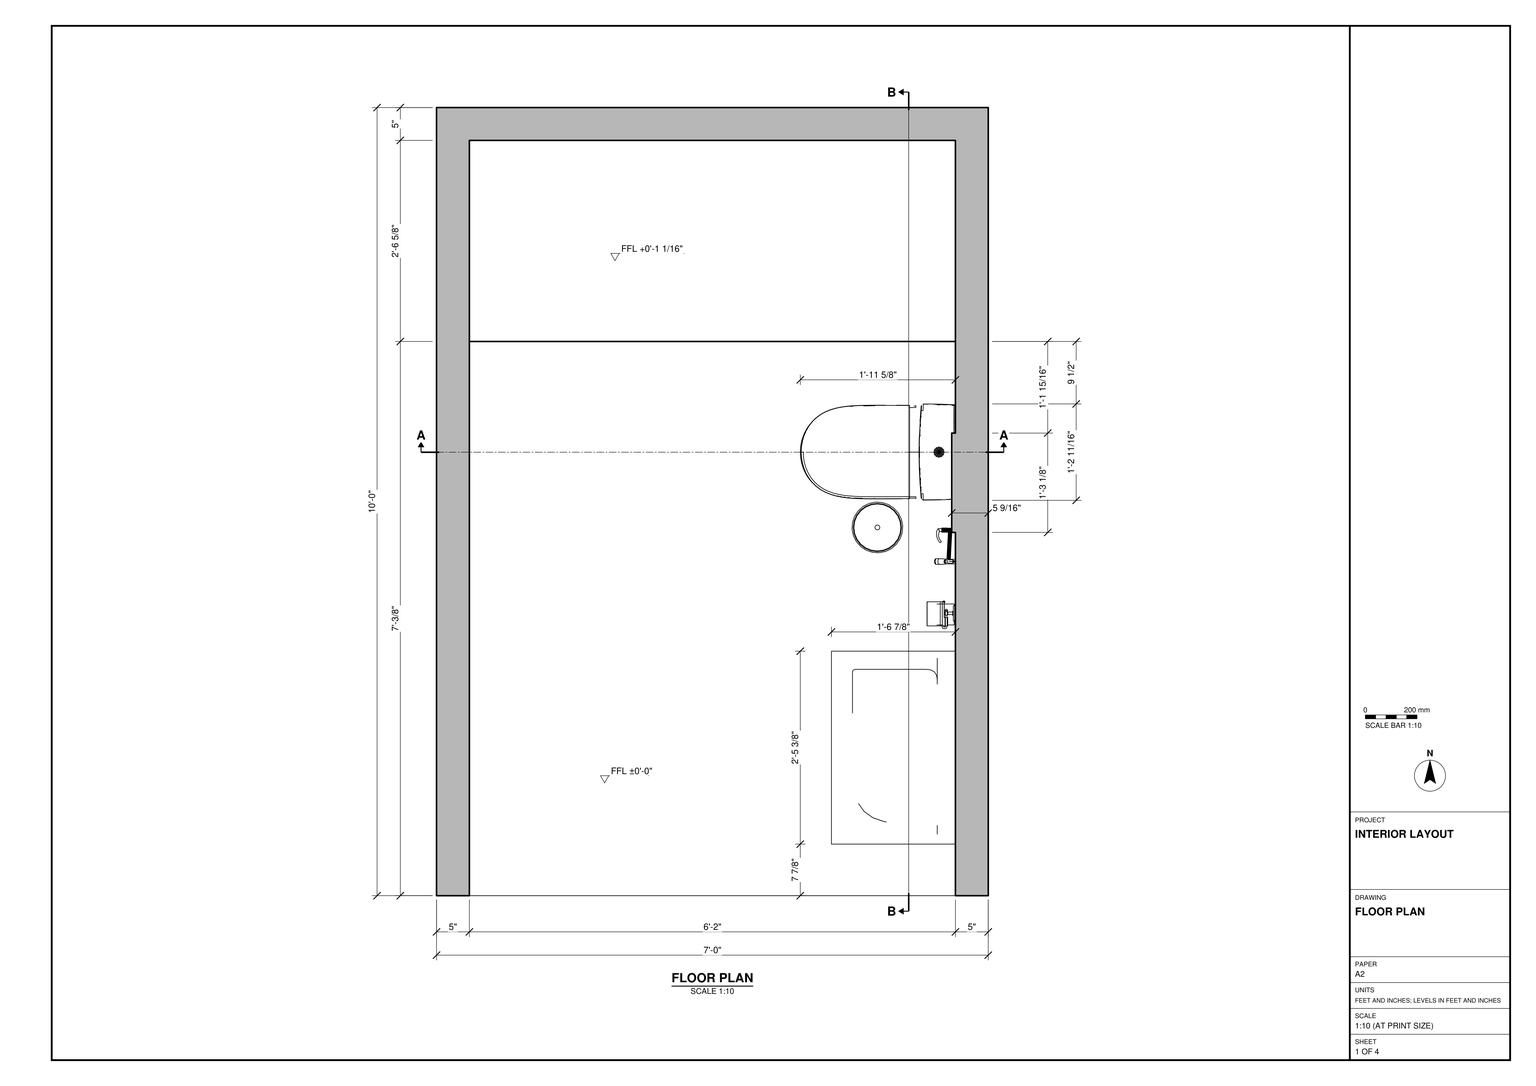
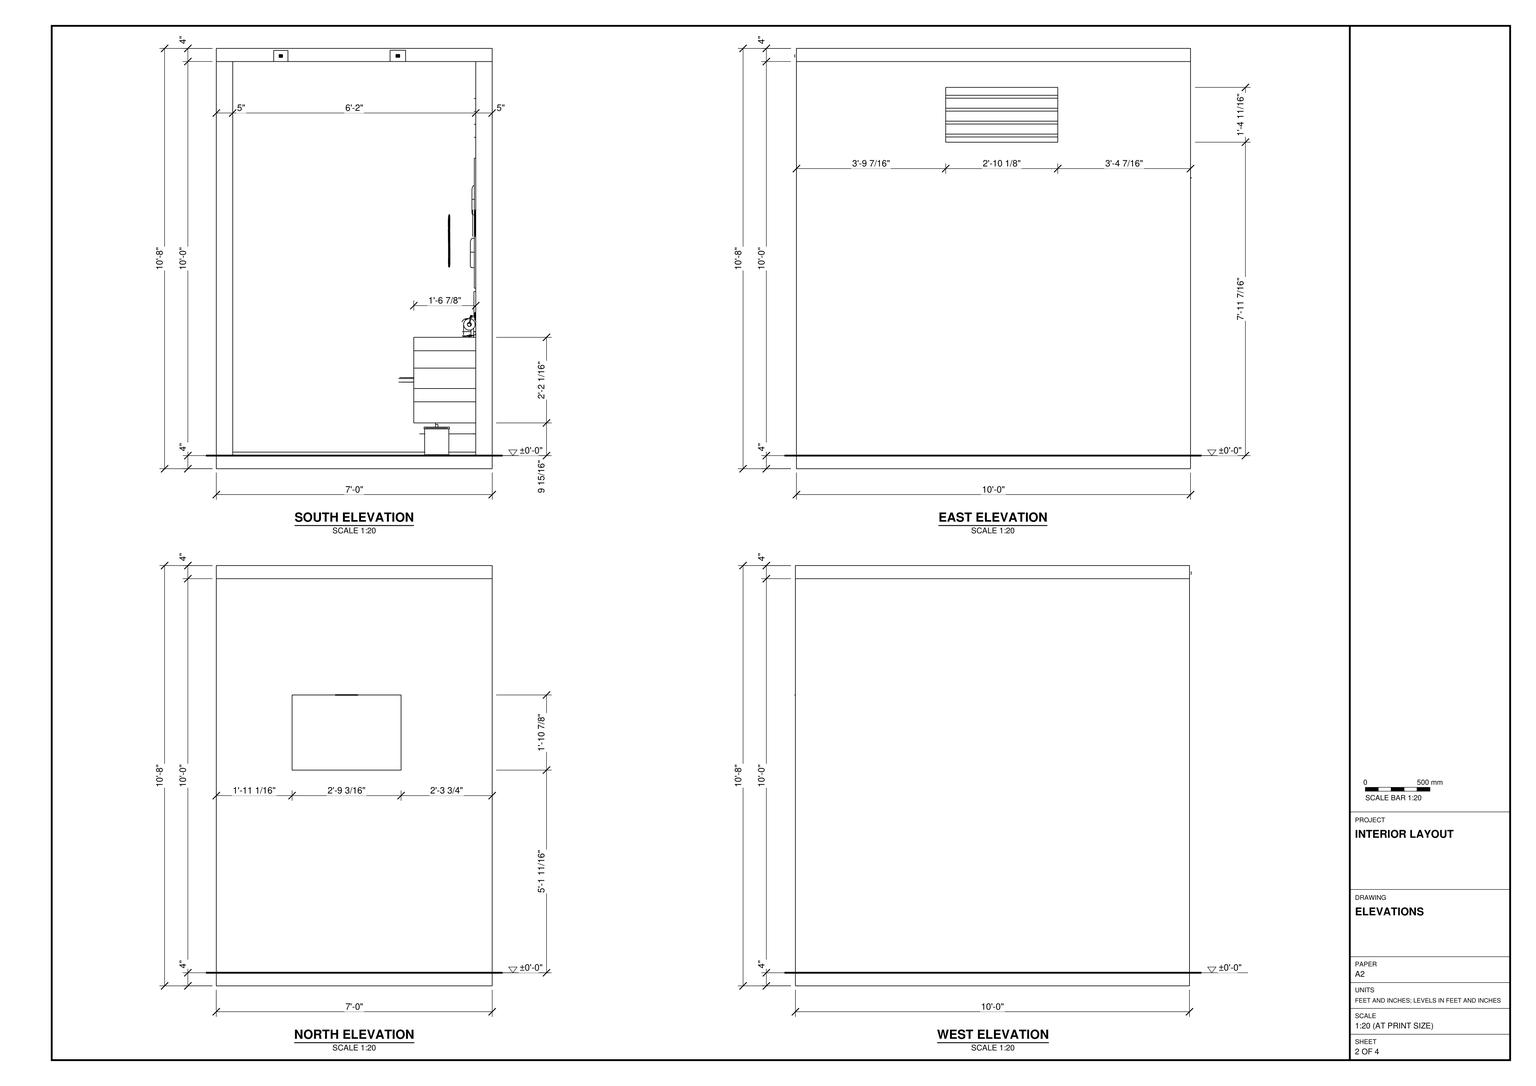
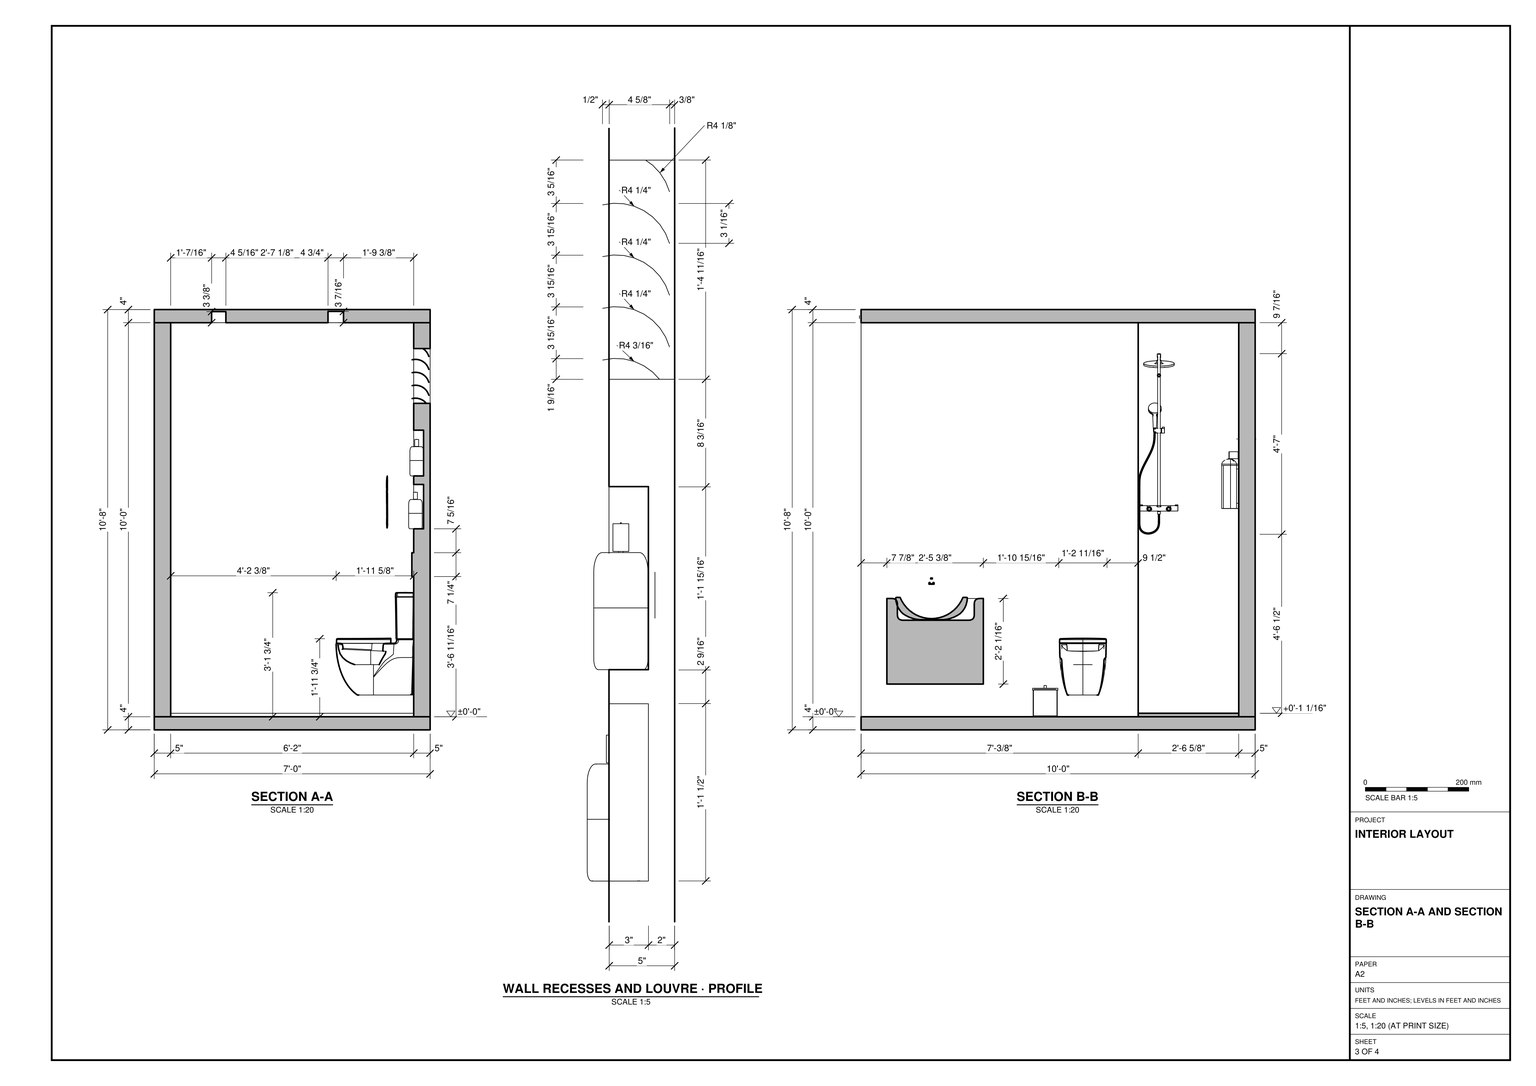
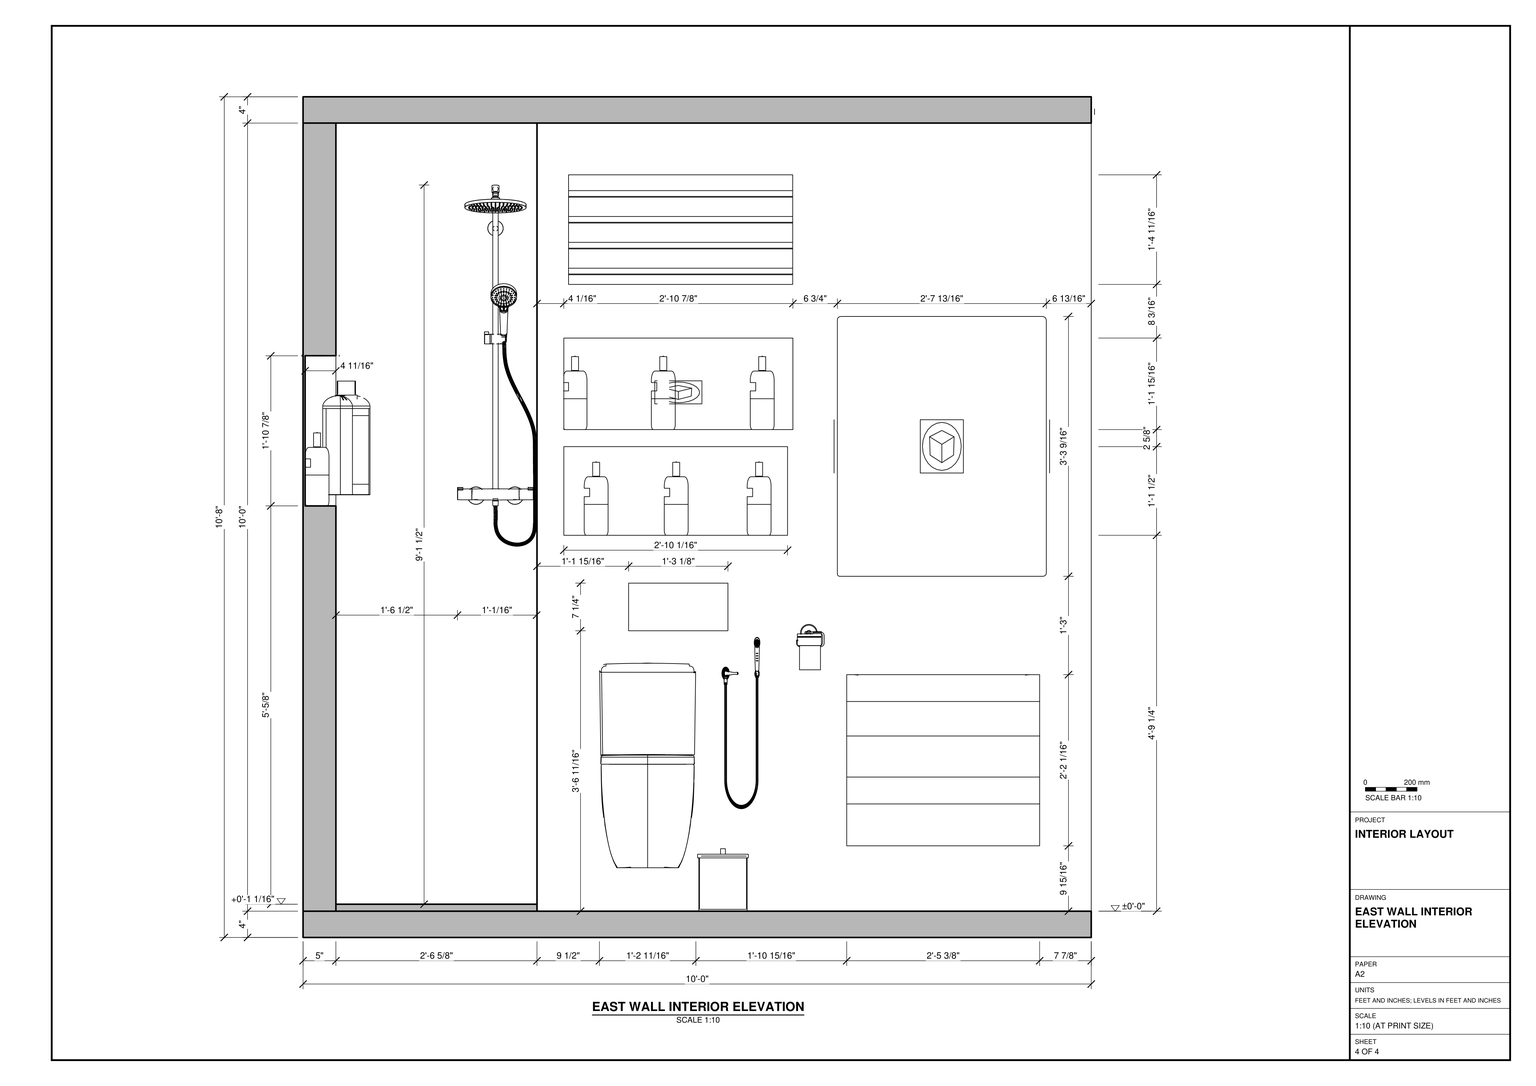
Build the bathroom in SketchUp from task_files/diagram_01.pdf. Work in feet and inches. The room is 7'-0" wide east to west, 10'-0" long north to south and 10'-8" high overall. Use ±0'-0" as the main finished floor level. Form the floor and ceiling with 4" slabs and the north, east and west walls with 5" thicknesses. Leave the south end open as drawn.

At the north end, raise the shower floor to +0'-1 1/16" and place the screen along its south edge. Use section B-B to position the shower head, hand shower and controls. Along the east wall, place the wall-hung vanity and basin nearest the open end, then the toilet between the basin and shower. Include the basin tap, the hand spray beside the toilet and the bin. Follow the elevations for the north-wall opening and the high east-wall louvre, and use the enlarged section to form the wall recesses below the louvre.

Keep the walls, slabs, fixtures and each joinery piece in separate groups or components, and use components for repeated parts. Decor and loose items may be any suitable library components. Save one SketchUp model as output_files/bathroom_with_a_raised_shower_and_wall_hung_vanity.skp.

# SketchUp Ruby script. Lengths in inches.
U = 1.inch
M = Sketchup.active_model
def pt(a) = Geom::Point3d.new(a.map { |v| v * U })
def face(e, loops, mat)
  f = e.add_face(loops[0].map { |a| pt(a) })
  loops[1..].each { |l| e.add_face(l.map { |a| pt(a) }).erase! }
  f.material = f.back_material = mat if mat
  f
end
# faces: each face lists its corners as indices into pts; further lists are holes
def faces(e, pts, list, mat = nil) = list.each { |f| face(e, (f[0].is_a?(Array) ? f : [f]).map { |l| l.map { |i| pts[i] } }, mat) }
# xy, xz, yz: faces in a plane at the given z, y or x. An outline is a flat list of corners, or four numbers for a rectangle; further outlines are holes
def ring(l) = l.size == 4 ? [[l[0], l[1]], [l[2], l[1]], [l[2], l[3]], [l[0], l[3]]] : l.each_slice(2).to_a
def flat(e, list, mat, &to3) = list.each { |f| face(e, (f[0].is_a?(Array) ? f : [f]).map { |l| ring(l).map { |u, v| to3.(u, v) } }, mat) }
def xy(e, z, list, mat = nil) = flat(e, list, mat) { |x, y| [x, y, z] }
def xz(e, y, list, mat = nil) = flat(e, list, mat) { |x, z| [x, y, z] }
def yz(e, x, list, mat = nil) = flat(e, list, mat) { |y, z| [x, y, z] }
def lines(e, pts, list) = list.each { |a, b| e.add_line(pt(pts[a]), pt(pts[b])) }
# prism: a flat outline (further loops are holes) pulled along v
def prism(e, loops, v, mat = nil)
  f = face(e, loops, mat); d = Geom::Vector3d.new(v.map { |x| x * U })
  f.pushpull(f.normal.samedirection?(d) ? d.length : -d.length)
end
def box(e, o, s, mat = nil) = prism(e, [[o, [o[0] + s[0], o[1], o[2]], [o[0] + s[0], o[1] + s[1], o[2]], [o[0], o[1] + s[1], o[2]]]], [0, 0, s[2]], mat)
def at(x, y, z, deg = 0) = Geom::Transformation.translation(pt([x, y, z])) * Geom::Transformation.rotation(ORIGIN, Z_AXIS, deg.degrees)
def axes(o, x, y, z) = Geom::Transformation.new([*x, 0, *y, 0, *z, 0, *pt(o).to_a, 1])
def part(name) = M.definitions.add(name)
# library, detail: a bought-in or finely detailed component or shape, given as its bounding box
def library(name, o, s) = part(name).tap { |d| box(d.entities, o, s) }
def detail(e, o, s) = box(e.add_group.entities, o, s)
def put(e, d, t, mat = nil) = e.add_instance(d, t).tap { |i| i.material = mat if mat }
def group(e, t, mat = nil) = e.add_group.tap { |g| g.transformation = t; g.material = mat if mat }.entities
root = M.entities
M.materials.add("ESPELHO1").color = [192, 192, 192]
M.materials.add("[0011_Seashell]").color = [255, 245, 238]
M.materials.add("[Herringbone]").color = [130, 130, 130]
M.materials.add("[Square Glass Tile 02]").color = [120, 183, 140]
M.materials.add("[Square Glass Tile 03]").color = [160, 163, 141]
M.materials.add("[Tile Various Tan]").color = [214, 196, 169]
M.materials.add("[Translucent Glass Tinted]").color = [8, 201, 241]
M.materials["[Translucent Glass Tinted]"].alpha = 0.48
c1 = library("Inodoro ROCA Meridian-N compact",[-14.68,0,0],[14.68,23.62,31.16])
c2 = library("00230906_3D_ducha_hig.dwg\#1",[121.96,-107.5,-116.36],[35.26,104.03,274.49])
c3 = part("LIXEIRA INOX DE BANHEIRO")
g1 = group(c3.entities,at(-3.9375,-3.9375,0),"ESPELHO1")
xy(g1,0,[[3.9375,0,2.92,0.13,1.97,0.53,1.15,1.15,0.53,1.97,0.13,2.92,0,3.9375,0.13,4.96,0.53,5.91,1.15,6.72,1.97,7.35,2.92,7.74,3.9375,7.875,4.96,7.74,5.91,7.35,6.72,6.72,7.35,5.91,7.74,4.96,7.875,3.9375,7.74,2.92,7.35,1.97,6.72,1.15,5.91,0.53,4.96,0.13]])
xy(g1,0.39,[[3.9375,0.12,4.93,0.25,5.85,0.63,6.64,1.24,7.24,2.03,7.625,2.95,7.75,3.9375,7.625,4.93,7.24,5.85,6.64,6.64,5.85,7.24,4.93,7.625,3.9375,7.75,2.95,7.625,2.03,7.24,1.24,6.64,0.63,5.85,0.25,4.93,0.12,3.9375,0.25,2.95,0.63,2.03,1.24,1.24,2.03,0.63,2.95,0.25]])
xy(g1,11.8125,[[[3.9375,0,4.96,0.13,5.91,0.53,6.72,1.15,7.35,1.97,7.74,2.92,7.875,3.9375,7.74,4.96,7.35,5.91,6.72,6.72,5.91,7.35,4.96,7.74,3.9375,7.875,2.92,7.74,1.97,7.35,1.15,6.72,0.53,5.91,0.13,4.96,0,3.9375,0.13,2.92,0.53,1.97,1.15,1.15,1.97,0.53,2.92,0.13],[3.9375,0.12,2.95,0.25,2.03,0.63,1.24,1.24,0.63,2.03,0.25,2.95,0.12,3.9375,0.25,4.93,0.63,5.85,1.24,6.64,2.03,7.24,2.95,7.625,3.9375,7.75,4.93,7.625,5.85,7.24,6.64,6.64,7.24,5.85,7.625,4.93,7.75,3.9375,7.625,2.95,7.24,2.03,6.64,1.24,5.85,0.63,4.93,0.25]]])
p = [[2.92,0.13,0],[3.9375,0,0],[3.9375,0,11.8125],[2.92,0.13,11.8125],[4.96,0.13,0],[4.96,0.13,11.8125],
  [1.97,0.53,0],[1.97,0.53,11.8125],[5.91,0.53,0],[5.91,0.53,11.8125],[1.15,1.15,0],[1.15,1.15,11.8125],
  [6.72,1.15,0],[6.72,1.15,11.8125],[0.53,1.97,0],[0.53,1.97,11.8125],[7.35,1.97,0],[7.35,1.97,11.8125],
  [0.13,2.92,0],[0.13,2.92,11.8125],[7.74,2.92,0],[7.74,2.92,11.8125],[0,3.9375,0],[0,3.9375,11.8125],
  [7.875,3.9375,0],[7.875,3.9375,11.8125],[0.13,4.96,0],[0.13,4.96,11.8125],[7.74,4.96,0],[7.74,4.96,11.8125],
  [0.53,5.91,0],[0.53,5.91,11.8125],[7.35,5.91,0],[7.35,5.91,11.8125],[1.15,6.72,0],[1.15,6.72,11.8125],
  [6.72,6.72,0],[6.72,6.72,11.8125],[1.97,7.35,0],[1.97,7.35,11.8125],[5.91,7.35,0],[5.91,7.35,11.8125],
  [2.92,7.74,0],[2.92,7.74,11.8125],[4.96,7.74,0],[4.96,7.74,11.8125],[3.9375,7.875,0],[3.9375,7.875,11.8125],
  [2.95,0.25,11.8125],[3.9375,0.12,11.8125],[3.9375,0.12,0.39],[2.95,0.25,0.39],[4.93,0.25,11.8125],[4.93,0.25,0.39],
  [2.03,0.63,11.8125],[2.03,0.63,0.39],[5.85,0.63,11.8125],[5.85,0.63,0.39],[1.24,1.24,11.8125],[1.24,1.24,0.39],
  [6.64,1.24,11.8125],[6.64,1.24,0.39],[0.63,2.03,11.8125],[0.63,2.03,0.39],[7.24,2.03,11.8125],[7.24,2.03,0.39],
  [0.25,2.95,11.8125],[0.25,2.95,0.39],[7.625,2.95,11.8125],[7.625,2.95,0.39],[0.12,3.9375,11.8125],[0.12,3.9375,0.39],
  [7.75,3.9375,11.8125],[7.75,3.9375,0.39],[0.25,4.93,11.8125],[0.25,4.93,0.39],[7.625,4.93,11.8125],[7.625,4.93,0.39],
  [0.63,5.85,11.8125],[0.63,5.85,0.39],[7.24,5.85,11.8125],[7.24,5.85,0.39],[1.24,6.64,11.8125],[1.24,6.64,0.39],
  [6.64,6.64,11.8125],[6.64,6.64,0.39],[2.03,7.24,11.8125],[2.03,7.24,0.39],[5.85,7.24,11.8125],[5.85,7.24,0.39],
  [2.95,7.625,11.8125],[2.95,7.625,0.39],[4.93,7.625,11.8125],[4.93,7.625,0.39],[3.9375,7.75,11.8125],[3.9375,7.75,0.39]]
faces(g1,p,[[0,1,2,3],[1,4,5,2],[6,0,3,7],[4,8,9,5],[10,6,7,11],[8,12,13,9],[14,10,11,15],[12,16,17,13],
  [18,14,15,19],[16,20,21,17],[22,18,19,23],[20,24,25,21],[26,22,23,27],[24,28,29,25],[30,26,27,31],[28,32,33,29],
  [34,30,31,35],[32,36,37,33],[38,34,35,39],[36,40,41,37],[42,38,39,43],[40,44,45,41],[46,42,43,47],[44,46,47,45],
  [48,49,50,51],[49,52,53,50],[54,48,51,55],[52,56,57,53],[58,54,55,59],[56,60,61,57],[62,58,59,63],[60,64,65,61],
  [66,62,63,67],[64,68,69,65],[70,66,67,71],[68,72,73,69],[74,70,71,75],[72,76,77,73],[78,74,75,79],[76,80,81,77],
  [82,78,79,83],[80,84,85,81],[86,82,83,87],[84,88,89,85],[90,86,87,91],[88,92,93,89],[94,90,91,95],[92,94,95,93]])
g2 = group(c3.entities,at(-4.13,-4.13,11.42),"ESPELHO1")
xy(g2,0,[[4.4,0,3.33,0.07,2.31,0.41,1.41,1.01,0.69,1.82,0.21,2.79,0,3.84,0.07,4.92,0.41,5.94,1.01,6.84,1.82,7.56,2.79,8.04,3.84,8.25,4.92,8.18,5.94,7.84,6.84,7.24,7.56,6.43,8.04,5.46,8.25,4.4,8.18,3.33,7.84,2.31,7.24,1.41,6.43,0.69,5.46,0.21]])
xy(g2,0.79,[[[4.4,0,5.46,0.21,6.43,0.69,7.24,1.41,7.84,2.31,8.18,3.33,8.25,4.4,8.04,5.46,7.56,6.43,6.84,7.24,5.94,7.84,4.92,8.18,3.84,8.25,2.79,8.04,1.82,7.56,1.01,6.84,0.41,5.94,0.07,4.92,0,3.84,0.21,2.79,0.69,1.82,1.41,1.01,2.31,0.41,3.33,0.07],[4.15,3.73,4.05,3.74,3.95,3.77,3.87,3.83,3.8,3.91,3.75,4,3.73,4.1,3.74,4.2,3.77,4.3,3.83,4.38,3.91,4.45,4,4.49,4.1,4.51,4.2,4.51,4.3,4.48,4.38,4.42,4.45,4.34,4.49,4.25,4.51,4.15,4.51,4.05,4.48,3.95,4.42,3.87,4.34,3.8,4.25,3.75]]])
xy(g2,1.97,[[4.15,3.73,4.25,3.75,4.34,3.8,4.42,3.87,4.48,3.95,4.51,4.05,4.51,4.15,4.49,4.25,4.45,4.34,4.38,4.42,4.3,4.48,4.2,4.51,4.1,4.51,4,4.49,3.91,4.45,3.83,4.38,3.77,4.3,3.74,4.2,3.73,4.1,3.75,4,3.8,3.91,3.87,3.83,3.95,3.77,4.05,3.74]])
xz(g2,4.51,[[4.1,0.79,4.2,1.97]])
yz(g2,4.51,[[4.05,0.79,4.15,1.97]])
p = [[3.33,0.07,0],[4.4,0,0],[4.4,0,0.79],[3.33,0.07,0.79],[5.46,0.21,0],[5.46,0.21,0.79],
  [2.31,0.41,0],[2.31,0.41,0.79],[6.43,0.69,0],[6.43,0.69,0.79],[1.41,1.01,0],[1.41,1.01,0.79],
  [7.24,1.41,0],[7.24,1.41,0.79],[0.69,1.82,0],[0.69,1.82,0.79],[7.84,2.31,0],[7.84,2.31,0.79],
  [0.21,2.79,0],[0.21,2.79,0.79],[8.18,3.33,0],[8.18,3.33,0.79],[0,3.84,0],[0,3.84,0.79],
  [8.25,4.4,0],[8.25,4.4,0.79],[0.07,4.92,0],[0.07,4.92,0.79],[8.04,5.46,0],[8.04,5.46,0.79],
  [0.41,5.94,0],[0.41,5.94,0.79],[7.56,6.43,0],[7.56,6.43,0.79],[1.01,6.84,0],[1.01,6.84,0.79],
  [6.84,7.24,0],[6.84,7.24,0.79],[1.82,7.56,0],[1.82,7.56,0.79],[5.94,7.84,0],[5.94,7.84,0.79],
  [2.79,8.04,0],[2.79,8.04,0.79],[4.92,8.18,0],[4.92,8.18,0.79],[3.84,8.25,0],[3.84,8.25,0.79],
  [4.05,3.74,0.79],[4.15,3.73,0.79],[4.15,3.73,1.97],[4.05,3.74,1.97],[3.95,3.77,0.79],[3.95,3.77,1.97],
  [4.25,3.75,0.79],[4.25,3.75,1.97],[3.8,3.91,0.79],[3.87,3.83,0.79],[3.87,3.83,1.97],[3.8,3.91,1.97],
  [4.34,3.8,0.79],[4.42,3.87,0.79],[4.42,3.87,1.97],[4.34,3.8,1.97],[3.75,4,0.79],[3.75,4,1.97],
  [4.48,3.95,0.79],[4.48,3.95,1.97],[3.73,4.1,0.79],[3.73,4.1,1.97],[4.51,4.05,0.79],[4.51,4.05,1.97],
  [3.74,4.2,0.79],[3.74,4.2,1.97],[3.77,4.3,0.79],[3.77,4.3,1.97],[4.51,4.15,0.79],[4.49,4.25,0.79],
  [4.49,4.25,1.97],[4.51,4.15,1.97],[3.83,4.38,0.79],[3.83,4.38,1.97],[4.45,4.34,0.79],[4.38,4.42,0.79],
  [4.38,4.42,1.97],[4.45,4.34,1.97],[3.91,4.45,0.79],[3.91,4.45,1.97],[4,4.49,0.79],[4,4.49,1.97],
  [4.3,4.48,0.79],[4.3,4.48,1.97],[4.1,4.51,0.79],[4.1,4.51,1.97],[4.2,4.51,0.79],[4.2,4.51,1.97]]
faces(g2,p,[[0,1,2,3],[1,4,5,2],[6,0,3,7],[4,8,9,5],[10,6,7,11],[8,12,13,9],[14,10,11,15],[12,16,17,13],
  [18,14,15,19],[16,20,21,17],[22,18,19,23],[20,24,25,21],[26,22,23,27],[24,28,29,25],[30,26,27,31],[28,32,33,29],
  [34,30,31,35],[32,36,37,33],[38,34,35,39],[36,40,41,37],[42,38,39,43],[40,44,45,41],[46,42,43,47],[44,46,47,45],
  [48,49,50,51],[52,48,51,53],[49,54,55,50],[56,57,58,59],[57,52,53,58],[60,61,62,63],[54,60,63,55],[64,56,59,65],
  [61,66,67,62],[68,64,65,69],[66,70,71,67],[72,68,69,73],[74,72,73,75],[76,77,78,79],[80,74,75,81],[82,83,84,85],
  [77,82,85,78],[86,80,81,87],[88,86,87,89],[83,90,91,84],[92,88,89,93],[90,94,95,91]])
c4 = part("tampa\#1")
xy(c4.entities,0,[[[54.33,0,40.27,1.85,27.17,7.28,15.91,15.91,7.28,27.17,1.85,40.27,0,54.33,1.85,68.39,7.28,81.5,15.91,92.75,27.17,101.38,40.27,106.81,54.33,108.66,68.39,106.81,81.5,101.38,92.75,92.75,101.38,81.5,106.81,68.39,107.57,62.6,108.66,54.33,106.81,40.27,101.38,27.17,92.75,15.91,81.5,7.28,68.39,1.85],[54.33,3.23,67.56,4.97,79.88,10.08,90.46,18.2,98.58,28.78,103.6875,41.11,105.43,54.33,104.4,62.18,103.6875,67.56,98.58,79.88,90.46,90.46,79.88,98.58,67.56,103.6875,54.33,105.43,41.11,103.6875,28.78,98.58,18.2,90.46,10.08,79.88,4.97,67.56,3.23,54.33,4.97,41.11,10.08,28.78,18.2,18.2,28.78,10.08,41.11,4.97]]],"[0011_Seashell]")
xy(c4.entities,94.09,[[54.33,0,68.39,1.85,81.5,7.28,82.75,8.24,80.8,10.78,79.88,10.08,67.56,4.97,54.33,3.23,41.11,4.97,28.78,10.08,27.87,10.78,25.92,8.24,27.17,7.28,40.27,1.85],[18.2,14.16,20.15,16.7,18.2,18.2],[90.46,14.16,90.46,18.2,88.51,16.7]],"[0011_Seashell]")
xy(c4.entities,118.11,[[18.2,14.16,18.2,18.2,10.08,28.78,4.97,41.11,3.23,54.33,4.97,67.56,10.08,79.88,18.2,90.46,28.78,98.58,41.11,103.6875,54.33,105.43,67.56,103.6875,79.88,98.58,90.46,90.46,98.58,79.88,103.6875,67.56,104.4,62.18,105.43,54.33,103.6875,41.11,98.58,28.78,90.46,18.2,90.46,14.16,92.75,15.91,101.38,27.17,106.81,40.27,108.66,54.33,107.57,62.6,106.81,68.39,101.38,81.5,92.75,92.75,81.5,101.38,68.39,106.81,54.33,108.66,40.27,106.81,27.17,101.38,15.91,92.75,7.28,81.5,1.85,68.39,0,54.33,1.85,40.27,7.28,27.17,15.91,15.91],[18.2,18.2,18.2,90.46,10.08,79.88,4.97,67.56,3.23,54.33,4.97,41.11,10.08,28.78],[90.46,18.2,98.58,28.78,103.6875,41.11,105.43,54.33,104.4,62.18,103.6875,67.56,98.58,79.88,90.46,90.46]],"[0011_Seashell]")
xy(c4.entities,121.26,[[18.2,18.2,18.2,90.46,10.08,79.88,4.97,67.56,3.23,54.33,4.97,41.11,10.08,28.78]],"[0011_Seashell]")
p = [[40.27,1.85,0],[54.33,0,0],[54.33,0,94.09],[40.27,1.85,94.09],[68.39,1.85,0],[68.39,1.85,94.09],
  [27.17,7.28,0],[27.17,7.28,94.09],[81.5,7.28,0],[81.5,7.28,94.09],[54.33,3.23,0],[41.11,4.97,0],
  [41.11,4.97,94.09],[54.33,3.23,94.09],[67.56,4.97,0],[67.56,4.97,94.09],[28.78,10.08,0],[28.78,10.08,94.09],
  [79.88,10.08,0],[79.88,10.08,94.09],[26.02,8.15,94.08],[25.92,8.24,94.09],[24.89,9.02,94.26],[23.79,9.87,94.63],
  [22.74,10.67,95.19],[21.76,11.43,95.93],[20.87,12.11,96.83],[20.09,12.71,97.875],[19.42,13.22,99.05],[18.9,13.625,100.32],
  [18.51,13.92,101.68],[18.28,14.1,103.08],[18.2,14.16,104.52],[18.2,14.16,118.11],[15.91,15.91,118.11],[15.91,15.91,0],
  [90.46,14.16,118.11],[90.46,14.16,104.52],[90.38,14.1,103.08],[90.15,13.92,101.68],[89.77,13.625,100.32],[89.24,13.22,99.05],
  [88.57,12.71,97.875],[87.79,12.11,96.83],[86.9,11.43,95.93],[85.92,10.67,95.19],[84.87,9.87,94.63],[83.77,9.02,94.26],
  [82.75,8.24,94.09],[82.64,8.15,94.08],[92.75,15.91,0],[92.75,15.91,118.11],[18.2,18.2,0],[18.2,18.2,94.09],
  [20.15,16.7,94.09],[27.87,10.78,94.09],[90.46,18.2,0],[80.8,10.78,94.09],[88.51,16.7,94.09],[90.46,18.2,94.09],
  [7.28,27.17,0],[7.28,27.17,118.11],[101.38,27.17,0],[101.38,27.17,118.11],[10.08,28.78,0],[10.08,28.78,118.11],
  [18.2,18.2,118.11],[90.46,18.2,118.11],[98.58,28.78,118.11],[98.58,28.78,0],[1.85,40.27,0],[1.85,40.27,118.11],
  [106.81,40.27,0],[106.81,40.27,118.11],[4.97,41.11,0],[4.97,41.11,118.11],[103.6875,41.11,0],[103.6875,41.11,118.11],
  [0,54.33,0],[0,54.33,118.11],[108.66,54.33,0],[108.66,54.33,118.11],[3.23,54.33,0],[3.23,54.33,118.11],
  [105.43,54.33,0],[105.43,54.33,118.11],[1.85,68.39,0],[1.85,68.39,118.11],[4.97,67.56,0],[4.97,67.56,118.11],
  [104.4,62.18,0],[104.4,62.18,118.11],[107.57,62.6,0],[107.57,62.6,118.11],[103.6875,67.56,0],[103.6875,67.56,118.11],
  [106.81,68.39,0],[106.81,68.39,118.11],[10.08,79.88,0],[10.08,79.88,118.11],[98.58,79.88,0],[98.58,79.88,118.11],
  [7.28,81.5,0],[7.28,81.5,118.11],[101.38,81.5,0],[101.38,81.5,118.11],[18.2,90.46,0],[18.2,90.46,118.11],
  [90.46,90.46,0],[90.46,90.46,118.11],[15.91,92.75,0],[15.91,92.75,118.11],[92.75,92.75,0],[92.75,92.75,118.11],
  [28.78,98.58,0],[28.78,98.58,118.11],[79.88,98.58,0],[79.88,98.58,118.11],[27.17,101.38,0],[27.17,101.38,118.11],
  [81.5,101.38,0],[81.5,101.38,118.11],[41.11,103.6875,0],[41.11,103.6875,118.11],[67.56,103.6875,0],[67.56,103.6875,118.11],
  [40.27,106.81,0],[40.27,106.81,118.11],[68.39,106.81,0],[68.39,106.81,118.11],[54.33,105.43,0],[54.33,105.43,118.11],
  [54.33,108.66,0],[54.33,108.66,118.11],[54.33,3.23,117.72],[41.11,4.97,117.72],[67.56,4.97,117.72],[28.78,10.08,117.72],
  [79.88,10.08,117.72],[26.84,11.57,94.26],[81.82,11.57,94.26],[20.15,16.7,117.72],[20.15,16.7,104.52],[20.23,16.64,103.08],
  [20.46,16.46,101.68],[20.85,16.17,100.32],[21.375,15.76,99.05],[22.04,15.25,97.875],[22.82,14.65,96.83],[23.71,13.97,95.93],
  [24.69,13.22,95.19],[25.74,12.41,94.63],[88.43,16.64,103.08],[88.51,16.7,104.52],[88.51,16.7,117.72],[82.92,12.41,94.63],
  [83.97,13.22,95.19],[84.95,13.97,95.93],[85.84,14.65,96.83],[86.625,15.25,97.875],[87.29,15.76,99.05],[87.82,16.17,100.32],
  [88.2,16.46,101.68],[42.12,27.39,117.71],[36.2,25.67,117.71],[30.52,23.3,117.71],[25.15,20.29,117.71],[54.33,28.78,117.71],
  [48.18,28.43,117.71],[72.46,25.67,117.71],[66.55,27.39,117.71],[60.48,28.43,117.71],[83.51,20.29,117.71],[78.14,23.3,117.71],
  [18.2,18.2,121.26],[28.78,98.58,121.26],[18.2,90.46,121.26],[90.46,90.46,121.26],[90.46,18.2,120.87],[79.88,98.58,121.26],
  [41.11,103.6875,121.26],[67.56,103.6875,121.26],[54.33,105.43,121.26],[10.08,28.78,121.26],[98.34,28.84,122.46],[4.97,41.11,121.26],
  [103.39,41.18,122.94],[3.23,54.33,121.26],[105.25,54.38,122.29],[4.97,67.56,121.26],[104.4,62.18,121.26],[103.6875,67.56,121.26],
  [10.08,79.88,121.26],[98.58,79.88,121.26]]
faces(c4.entities,p,[[0,1,2,3],[1,4,5,2],[6,0,3,7],[4,8,9,5],[10,11,12,13],[14,10,13,15],[11,16,17,12],[18,14,15,19],
  [20,21,22,23,24,25,26,27,28,29,30,31,32,33,34,35,6,7],[36,37,38,39,40,41,42,43,44,45,46,47,48,49,9,8,50,51],[16,52,53,54,55,17],[56,18,19,57,58,59],[60,35,34,61],[50,62,63,51],[52,64,65,66,53],[67,68,69,56,59],
  [70,60,61,71],[62,72,73,63],[64,74,75,65],[76,69,68,77],[78,70,71,79],[72,80,81,73],[74,82,83,75],[84,76,77,85],
  [86,78,79,87],[82,88,89,83],[90,84,85,91],[80,92,93,81],[94,90,91,95],[92,96,97,93],[88,98,99,89],[100,94,95,101],
  [102,86,87,103],[96,104,105,97],[98,106,107,99],[108,100,101,109],[110,102,103,111],[104,112,113,105],[106,114,115,107],[116,108,109,117],
  [118,110,111,119],[112,120,121,113],[114,122,123,115],[124,116,117,125],[126,118,119,127],[120,128,129,121],[122,130,131,123],[130,124,125,131],
  [132,126,127,133],[128,132,133,129],[13,134,135,12],[15,136,134,13],[12,135,137,17],[19,138,136,15],[7,21,20],[48,9,49],
  [22,21,55,139],[48,47,140,57],[17,137,141,142,143,144,145,146,147,148,149,150,151,139,55],[152,153,154,138,19,57,140,155,156,157,158,159,160,161,162],[53,66,141,142,54],[58,153,154,67,59],[23,22,139,151],[47,46,155,140],
  [24,23,151,150],[46,45,156,155],[25,24,150,149],[45,44,157,156],[26,25,149,148],[44,43,158,157],[27,26,148,147],[43,42,159,158],
  [28,27,147,146],[42,41,160,159],[29,28,146,145],[41,40,161,160],[30,29,145,144],[40,39,162,161],[31,30,144,143],[39,38,152,162],
  [32,31,143,142],[38,37,153,152],[32,142,141,33],[36,154,153,37],[137,135,134,163,164,165,166,141],[134,123,135],[123,134,136,131],[163,134,167,168],
  [134,136,138,169,170,171,167],[135,123,137],[125,131,136],[138,125,136],[137,115,141],[123,115,137],[117,125,138],[169,138,154,172,173],
  [154,117,138],[141,66,33],[154,36,67],[115,107,141],[141,107,66],[66,141,174],[175,176,141],[141,176,174],
  [166,175,141],[109,117,154],[154,177,172],[67,109,154],[178,177,154],[67,178,154],[165,175,166],[172,179,173],
  [177,179,172],[180,175,165],[164,180,165],[173,179,169],[163,180,164],[169,181,170],[179,181,169],[182,180,163],
  [168,182,163],[170,181,171],[167,182,168],[181,182,171],[171,182,167],[174,183,65,66],[67,68,178],[184,178,68],
  [183,185,75,65],[186,184,77],[68,77,184],[185,187,83,75],[77,85,186],[188,186,85],[187,189,89,83],[85,91,188],
  [190,188,91],[91,95,191,190],[189,192,99,89],[95,101,193,191],[192,176,107,99],[101,109,177,193],[107,176,175,115],[117,179,177,109],
  [115,175,180,123],[125,181,179,117],[123,180,182,131],[131,182,181,125],[178,184,177],[193,177,184],[186,191,184],[191,193,184],
  [188,190,186],[190,191,186]],"[0011_Seashell]")
c5 = library("CONDI",[0,0,0],[334.65,157.48,859.19])
c6 = part("Condicionador")
put(c6.entities,c4,at(112.99,24.41,758.01),"[0011_Seashell]")
put(c6.entities,c5,at(0,0,0))
c7 = library("vidro",[0,0,0],[334.65,157.48,859.19])
c8 = library("Sans titre",[5.94,-9.89,0],[60.45,60.45,73.03])
c9 = library("Pocelanosa Basin Urban 55cm & Tap",[0,0,0],[21.84,16.54,13.4375])
c10 = library("16__hcb56766_dxf.dxf",[0,0,0],[12.11,18.43,55])
c11 = library("Group\#12",[-0.5,-0.5,-0.1],[34.1875,5.6875,0.2])
c12 = library("Group\#13",[-0.5,-0.5,0],[4,35.875,16.53])
c13 = library("Group\#10",[-0.5,-0.5,0],[5.34,116,3.375])
c14 = library("Group\#11",[-0.5,-0.5,0],[5.73,116,3.4375])
c15 = library("Group\#4",[-0.4375,-0.4375,0],[18.875,29.375,26.0625])
c16 = library("Group\#6",[-0.5,-0.5,0],[1.4375,32.8125,39.5625])
c17 = part("Group18\#1")
p = [[17.0625,-6.875,0.39],[-17.0625,-6.875,0.39],[-17.0625,-6.75,1.2],[17.0625,-6.75,1.2],[-17.0625,-6.79,2.01],[17.0625,-6.79,2.01],
  [-17.0625,-6.98,2.79],[17.0625,-6.98,2.79],[-17.0625,-7.32,3.53],[17.0625,-7.32,3.53],[-17.0625,-7.79,4.19],[17.0625,-7.79,4.19],
  [-17.0625,-8.34,4.72],[17.0625,-8.34,4.72]]
faces(c17.entities,p,[[0,1,2,3],[3,2,4,5],[5,4,6,7],[7,6,8,9],[9,8,10,11],[11,10,12,13]])
c18 = part("Group19\#1")
p = [[-17.0625,-2.82,1.2],[17.0625,-2.82,1.2],[17.0625,-2.9375,0.39],[-17.0625,-2.9375,0.39],[-17.0625,-2.85,2.01],[17.0625,-2.85,2.01],
  [-17.0625,-3.04,2.79],[17.0625,-3.04,2.79],[-17.0625,-3.38,3.53],[17.0625,-3.38,3.53],[-17.0625,-3.85,4.19],[17.0625,-3.85,4.19],
  [-17.0625,-4.4375,4.75],[17.0625,-4.4375,4.75],[-17.0625,-5.12,5.18],[17.0625,-5.12,5.18],[-17.0625,-5.875,5.48],[17.0625,-5.875,5.48]]
faces(c18.entities,p,[[0,1,2,3],[4,5,1,0],[6,7,5,4],[8,9,7,6],[10,11,9,8],[12,13,11,10],[14,15,13,12],[16,17,15,14]])
c19 = part("Group20\#1")
p = [[-17.0625,1.12,1.2],[17.0625,1.12,1.2],[17.0625,1,0.39],[-17.0625,1,0.39],[-17.0625,1.08,2.01],[17.0625,1.08,2.01],
  [-17.0625,0.9,2.79],[17.0625,0.9,2.79],[-17.0625,0.56,3.53],[17.0625,0.56,3.53],[-17.0625,0.09,4.19],[17.0625,0.09,4.19],
  [-17.0625,-0.5,4.75],[17.0625,-0.5,4.75],[-17.0625,-1.18,5.18],[17.0625,-1.18,5.18],[-17.0625,-1.9375,5.48],[17.0625,-1.9375,5.48]]
faces(c19.entities,p,[[0,1,2,3],[4,5,1,0],[6,7,5,4],[8,9,7,6],[10,11,9,8],[12,13,11,10],[14,15,13,12],[16,17,15,14]])
c20 = part("Group21\#1")
p = [[-17.0625,5.06,1.2],[17.0625,5.06,1.2],[17.0625,4.9375,0.39],[-17.0625,4.9375,0.39],[-17.0625,5.02,2.01],[17.0625,5.02,2.01],
  [-17.0625,4.83,2.79],[17.0625,4.83,2.79],[-17.0625,4.5,3.53],[17.0625,4.5,3.53],[-17.0625,4.03,4.19],[17.0625,4.03,4.19],
  [-17.0625,3.4375,4.75],[17.0625,3.4375,4.75],[-17.0625,2.75,5.18],[17.0625,2.75,5.18],[-17.0625,2,5.48],[17.0625,2,5.48]]
faces(c20.entities,p,[[0,1,2,3],[4,5,1,0],[6,7,5,4],[8,9,7,6],[10,11,9,8],[12,13,11,10],[14,15,13,12],[16,17,15,14]])
c21 = part("Group22\#1")
p = [[-17.0625,7.96,4.19],[17.0625,7.96,4.19],[17.0625,8.34,3.66],[-17.0625,8.34,3.66],[-17.0625,7.375,4.75],[17.0625,7.375,4.75],
  [-17.0625,6.69,5.18],[17.0625,6.69,5.18],[-17.0625,5.9375,5.48],[17.0625,5.9375,5.48]]
faces(c21.entities,p,[[0,1,2,3],[4,5,1,0],[6,7,5,4],[8,9,7,6]])
c22 = part("Group16\#1")
put(c22.entities,c17,at(0,0,0))
put(c22.entities,c18,at(0,0,0))
put(c22.entities,c19,at(0,0,0))
put(c22.entities,c20,at(0,0,0))
put(c22.entities,c21,at(0,0,0))
c23 = library("Grupo\#25",[0.45,21.05,9.1],[4.32,4.21,6.93])
xz(root,84.38,[[5,1.0625,79,120]],"[Translucent Glass Tinted]")
p = [[84,45.45,95.43],[84,45.45,112.12],[84,79.58,112.12],[84,79.58,95.43]]
lines(root,p,[[0,1],[1,2],[2,3],[3,0]])
put(root,c1,at(79,74.88,6.61,90))
put(root,c2,axes([90.79,50.25,26.67],[-0.09517,0,0],[0,-0.05567,0],[0,0,0.09517]))
put(root,c3,axes([67.11,56.0625,0],[-0.9353,0,0],[0,-0.9353,0],[0,0,0.71083]))
put(root,c6,axes([30.18,115,61.71],[0.027,0,0],[0,0.02794,0],[0,0,0.02017]))
put(root,c7,axes([43.88,113.34,63.39],[0.02738,-0.01259,0],[0.0127,0.02762,0],[0,0,0.02016]))
put(root,c8,axes([77.0625,74.15,57.23],[0.0682,0,0],[0,0.06015,0],[0,0,0.15326]))
put(root,c8,axes([76.9375,49.34,57.23],[0.0682,0,0],[0,0.06015,0],[0,0,0.15326]))
put(root,c8,axes([76.9375,61.97,57.23],[0.0682,0,0],[0,0.06015,0],[0,0,0.15326]))
put(root,c8,axes([77.4375,77.37,73.33],[0.0682,0,0],[0,0.06015,0],[0,0,0.15326]))
put(root,c8,axes([77.4375,63.93,73.33],[0.0682,0,0],[0,0.06015,0],[0,0,0.15326]))
put(root,c8,axes([77.4375,48.87,73.33],[0.0682,0,0],[0,0.06015,0],[0,0,0.15326]))
put(root,c8,axes([39.66,116.65,61.71],[0.0682,0,0],[0,0.06015,0],[0,0,0.15326]))
put(root,c9,at(61.27,32.37,28.82,-90))
put(root,c10,at(54.79,96.49,55.5625,-90))
g3 = group(root,at(0,0,0))
xy(g3,0,[[0,0,0,120,84,120,84,0,79,0,79,115,5,115,5,0]])
xy(g3,42.7,[[78.4375,55.3125,79,70.4375]])
xy(g3,49.95,[[78.4375,55.3125,79,70.4375]])
xy(g3,57.23,[[79,46.24,82,80.3]])
xy(g3,61.71,[[27.74,115,60.93,119.6875]])
xy(g3,73.33,[[79,45.42,82,80.3]])
xy(g3,95.43,[[79,45.45,84,79.58]])
xy(g3,112.12,[[79,45.45,84,79.58]])
xy(g3,120,[[0,0,5,0,5,115,79,115,79,0,84,0,84,120,0,120]])
xz(g3,0,[[0,0,5,120],[79,0,84,120]])
xz(g3,45.42,[[79,73.33,82,87.26]])
xz(g3,45.45,[[79,95.43,84,112.12]])
xz(g3,46.24,[[79,57.23,82,70.73]])
xz(g3,55.3125,[[78.4375,42.7,79,49.95]])
xz(g3,70.4375,[[78.4375,42.7,79,49.95]])
xz(g3,79.58,[[79,95.43,84,112.12]])
xz(g3,80.3,[[79,57.23,82,70.73],[79,73.33,82,87.26]])
xz(g3,115,[[5,0,79,1.0625]])
xz(g3,115,[[5,1.0625,79,60],[[5,60,79,120],[27.74,61.71,60.93,84.58]]],"[Tile Various Tan]")
xz(g3,119.6875,[[27.74,61.71,60.93,84.58]])
xz(g3,120,[[0,0,84,120]])
yz(g3,0,[[0,0,120,120]])
yz(g3,5,[[0,0,115,120]],"[Herringbone]")
yz(g3,27.74,[[115,61.71,119.6875,84.58]])
yz(g3,60.93,[[115,61.71,119.6875,84.58]])
yz(g3,78.4375,[[55.3125,42.7,70.4375,49.95]])
yz(g3,79,[[[0,0,115,120],[45.45,95.43,79.58,112.12],[45.42,73.33,80.3,87.26],[46.24,57.23,80.3,70.73],[55.3125,42.7,70.4375,49.95]]])
yz(g3,82,[[46.24,57.23,80.3,70.73],[45.42,73.33,80.3,87.26]])
yz(g3,84,[[[0,0,120,120],[45.45,95.43,79.58,112.12]]])
put(g3,c11,at(27.74,115,84.58))
put(g3,c12,at(79,45.42,70.73))
g4 = group(root,at(0,0,-4))
xy(g4,0,[[0,0,84,120]])
xy(g4,4,[[0,0,84,120]],"[Square Glass Tile 03]")
xz(g4,0,[[0,0,84,4]])
xz(g4,120,[[0,0,84,4]])
yz(g4,0,[[0,0,120,4]])
yz(g4,84,[[0,0,120,4]])
g5 = group(root,at(0,0,120))
xy(g5,0,[[0,0,0,120,84,120,84,0,57.63,0,57.63,115,52.9,115,52.9,0,21.81,0,21.81,115,17.47,115,17.47,0]])
xy(g5,4,[[0,0,84,120]])
xz(g5,0,[[0,0,17.47,0,17.47,3.375,21.81,3.375,21.81,0,52.9,0,52.9,3.4375,57.63,3.4375,57.63,0,84,0,84,4,0,4],[17.47,0,21.81,3.375],[52.9,0,57.63,3.4375]])
xz(g5,115,[[17.47,0,21.81,3.375],[52.9,0,57.63,3.4375]])
xz(g5,120,[[0,0,84,4]])
yz(g5,0,[[0,0,120,4]])
yz(g5,84,[[0,0,120,4]])
put(g5,c13,at(17.47,0,0))
put(g5,c14,at(52.9,0,0))
put(root,c15,at(60.5625,8.29,9.95))
put(root,c16,at(78.5625,6.84,50.99))
g6 = group(root,at(5,84.38,0))
box(g6,[0,0,0],[74,30.62,1.0625],"[Square Glass Tile 02]")
put(root,c22,axes([78.125,62.51,103.78],[0,1,0],[0,0,1],[1,0,0]))
put(root,c23,at(79.45,65.92,27.65,180))
